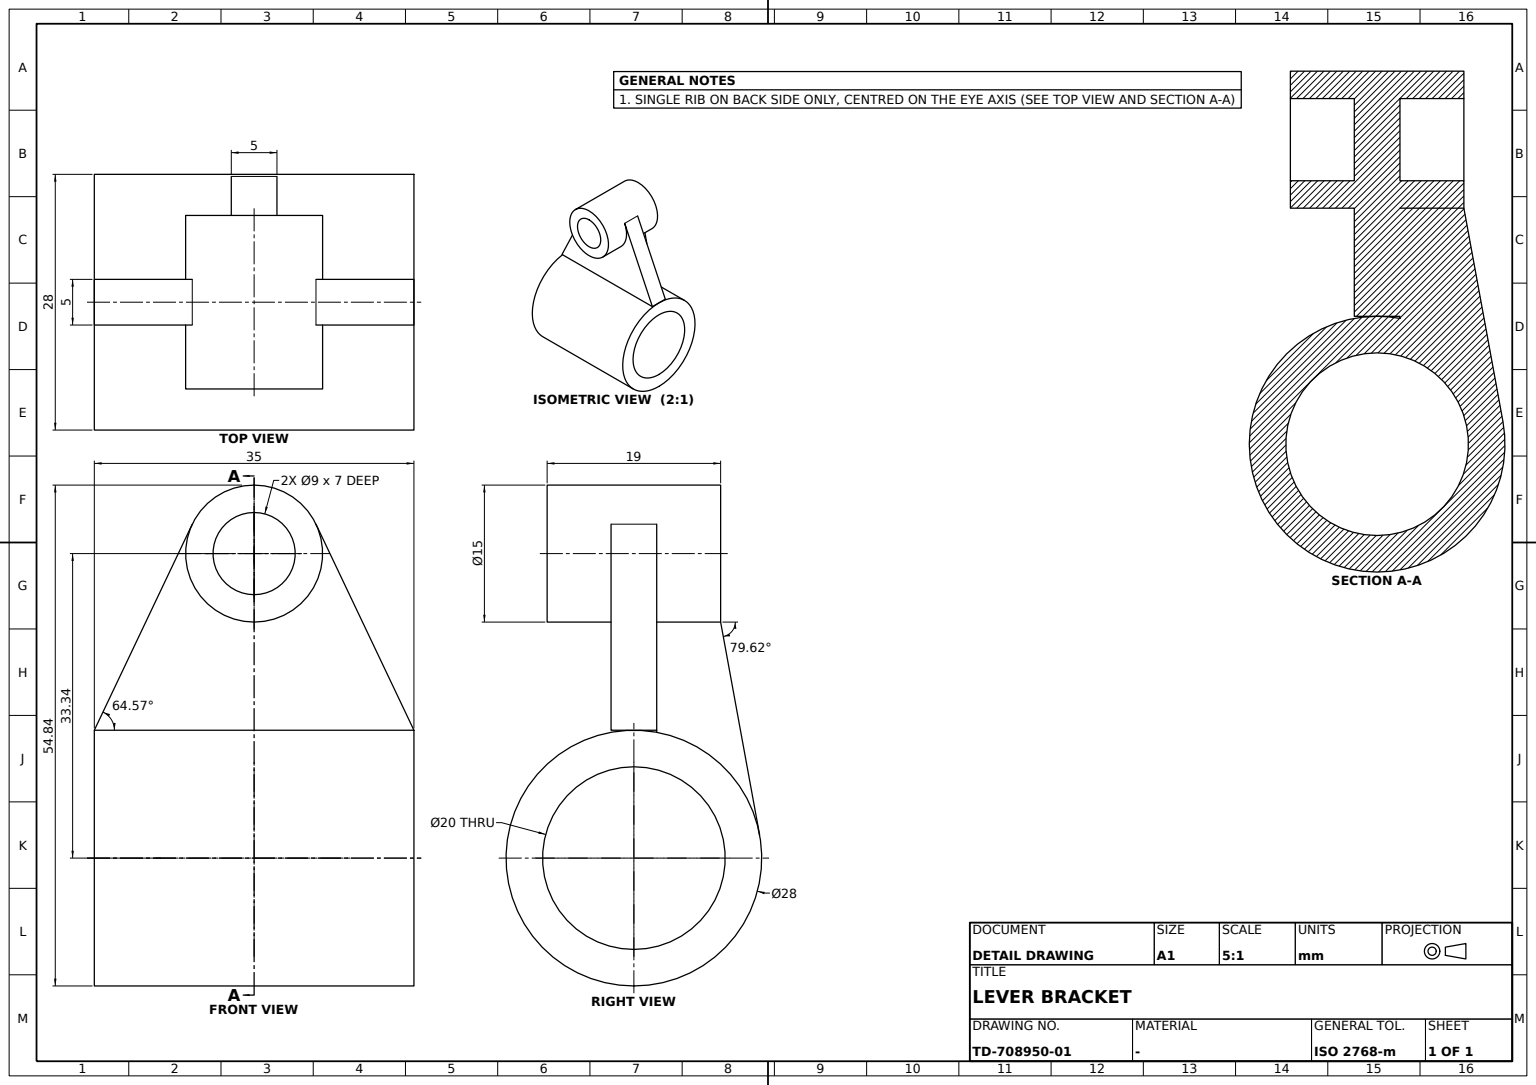
ISO-10303-21;
HEADER;
FILE_DESCRIPTION((''),'2;1');
FILE_NAME('','',(''),(''),'','','');
FILE_SCHEMA(('AUTOMOTIVE_DESIGN'));
ENDSEC;
DATA;
#1=APPLICATION_CONTEXT('');
#2=PRODUCT_CONTEXT('',#1,'mechanical');
#3=PRODUCT('','','',(#2));
#4=PRODUCT_DEFINITION_FORMATION('','',#3);
#5=PRODUCT_DEFINITION_CONTEXT('',#1,'design');
#6=PRODUCT_DEFINITION('','',#4,#5);
#7=PRODUCT_DEFINITION_SHAPE('','',#6);
#8=(LENGTH_UNIT()NAMED_UNIT(*)SI_UNIT(.MILLI.,.METRE.));
#9=(NAMED_UNIT(*)PLANE_ANGLE_UNIT()SI_UNIT($,.RADIAN.));
#10=(NAMED_UNIT(*)SI_UNIT($,.STERADIAN.)SOLID_ANGLE_UNIT());
#11=UNCERTAINTY_MEASURE_WITH_UNIT(LENGTH_MEASURE(0.005),#8,'distance_accuracy_value','');
#12=(GEOMETRIC_REPRESENTATION_CONTEXT(3)GLOBAL_UNCERTAINTY_ASSIGNED_CONTEXT((#11))GLOBAL_UNIT_ASSIGNED_CONTEXT((#8,#9,#10))REPRESENTATION_CONTEXT('',''));
#13=CARTESIAN_POINT('',(0.,2.5,37.842022));
#14=VERTEX_POINT('',#13);
#15=CARTESIAN_POINT('',(0.,2.5,33.342022));
#16=DIRECTION('',(0.,1.,0.));
#17=DIRECTION('',(0.,0.,1.));
#18=AXIS2_PLACEMENT_3D('',#15,#16,#17);
#19=CIRCLE('',#18,4.5);
#20=EDGE_CURVE('',#14,#14,#19,.T.);
#21=ORIENTED_EDGE('',*,*,#20,.F.);
#22=EDGE_LOOP('',(#21));
#23=FACE_BOUND('',#22,.T.);
#24=CARTESIAN_POINT('',(0.,9.5,37.842022));
#25=VERTEX_POINT('',#24);
#26=CARTESIAN_POINT('',(0.,9.5,33.342022));
#27=AXIS2_PLACEMENT_3D('',#26,#16,#17);
#28=CIRCLE('',#27,4.5);
#29=EDGE_CURVE('',#25,#25,#28,.T.);
#30=ORIENTED_EDGE('',*,*,#29,.T.);
#31=EDGE_LOOP('',(#30));
#32=FACE_BOUND('',#31,.T.);
#33=CARTESIAN_POINT('',(0.,0.,33.342022));
#34=DIRECTION('',(-1.,0.,0.));
#35=AXIS2_PLACEMENT_3D('',#33,#16,#34);
#36=CYLINDRICAL_SURFACE('',#35,4.5);
#37=ADVANCED_FACE('',(#23,#32),#36,.F.);
#38=CARTESIAN_POINT('',(17.5,0.,-10.));
#39=VERTEX_POINT('',#38);
#40=CARTESIAN_POINT('',(17.5,0.,0.));
#41=DIRECTION('',(1.,0.,0.));
#42=DIRECTION('',(0.,0.,-1.));
#43=AXIS2_PLACEMENT_3D('',#40,#41,#42);
#44=CIRCLE('',#43,10.);
#45=EDGE_CURVE('',#39,#39,#44,.T.);
#46=ORIENTED_EDGE('',*,*,#45,.T.);
#47=EDGE_LOOP('',(#46));
#48=FACE_BOUND('',#47,.T.);
#49=CARTESIAN_POINT('',(-17.5,0.,-10.));
#50=VERTEX_POINT('',#49);
#51=CARTESIAN_POINT('',(-17.5,0.,0.));
#52=AXIS2_PLACEMENT_3D('',#51,#41,#42);
#53=CIRCLE('',#52,10.);
#54=EDGE_CURVE('',#50,#50,#53,.T.);
#55=ORIENTED_EDGE('',*,*,#54,.F.);
#56=EDGE_LOOP('',(#55));
#57=FACE_BOUND('',#56,.T.);
#58=CARTESIAN_POINT('',(0.,0.,0.));
#59=AXIS2_PLACEMENT_3D('',#58,#41,#16);
#60=CYLINDRICAL_SURFACE('',#59,10.);
#61=ADVANCED_FACE('',(#48,#57),#60,.F.);
#62=CARTESIAN_POINT('',(2.5,2.5,14.));
#63=VERTEX_POINT('',#62);
#64=CARTESIAN_POINT('',(2.5,2.5,13.774977));
#65=VERTEX_POINT('',#64);
#66=CARTESIAN_POINT('',(2.5,2.5,0.));
#67=VECTOR('',#42,1000.);
#68=LINE('',#66,#67);
#69=EDGE_CURVE('',#63,#65,#68,.T.);
#70=ORIENTED_EDGE('',*,*,#69,.F.);
#71=CARTESIAN_POINT('',(-2.5,2.5,14.));
#72=VERTEX_POINT('',#71);
#73=CARTESIAN_POINT('',(0.,2.5,14.));
#74=VECTOR('',#34,1000.);
#75=LINE('',#73,#74);
#76=EDGE_CURVE('',#63,#72,#75,.T.);
#77=ORIENTED_EDGE('',*,*,#76,.T.);
#78=CARTESIAN_POINT('',(-2.5,2.5,13.774977));
#79=VERTEX_POINT('',#78);
#80=CARTESIAN_POINT('',(-2.5,2.5,0.));
#81=LINE('',#80,#67);
#82=EDGE_CURVE('',#72,#79,#81,.T.);
#83=ORIENTED_EDGE('',*,*,#82,.T.);
#84=VECTOR('',#41,1000.);
#85=LINE('',#78,#84);
#86=EDGE_CURVE('',#79,#65,#85,.T.);
#87=ORIENTED_EDGE('',*,*,#86,.T.);
#88=EDGE_LOOP('',(#70,#77,#83,#87));
#89=FACE_BOUND('',#88,.T.);
#90=CARTESIAN_POINT('',(0.,2.5,0.));
#91=AXIS2_PLACEMENT_3D('',#90,#16,#34);
#92=PLANE('',#91);
#93=ADVANCED_FACE('',(#89),#92,.F.);
#94=ORIENTED_EDGE('',*,*,#45,.F.);
#95=EDGE_LOOP('',(#94));
#96=FACE_BOUND('',#95,.T.);
#97=CARTESIAN_POINT('',(17.5,0.,-14.));
#98=VERTEX_POINT('',#97);
#99=CIRCLE('',#43,14.);
#100=EDGE_CURVE('',#98,#98,#99,.T.);
#101=ORIENTED_EDGE('',*,*,#100,.T.);
#102=EDGE_LOOP('',(#101));
#103=FACE_BOUND('',#102,.T.);
#104=AXIS2_PLACEMENT_3D('',#40,#41,#16);
#105=PLANE('',#104);
#106=ADVANCED_FACE('',(#96,#103),#105,.T.);
#107=CARTESIAN_POINT('',(-6.773482,-2.5,36.562261));
#108=VERTEX_POINT('',#107);
#109=CARTESIAN_POINT('',(-6.773482,2.5,36.562261));
#110=VERTEX_POINT('',#109);
#111=CARTESIAN_POINT('',(-6.773482,0.,36.562261));
#112=VECTOR('',#16,1000.);
#113=LINE('',#111,#112);
#114=EDGE_CURVE('',#108,#110,#113,.T.);
#115=ORIENTED_EDGE('',*,*,#114,.T.);
#116=CARTESIAN_POINT('',(-17.5,2.5,14.));
#117=VERTEX_POINT('',#116);
#118=CARTESIAN_POINT('',(-19.702619,2.5,9.366991));
#119=DIRECTION('',(0.429365223,0.,0.903130946));
#120=VECTOR('',#119,1000.);
#121=LINE('',#118,#120);
#122=EDGE_CURVE('',#117,#110,#121,.T.);
#123=ORIENTED_EDGE('',*,*,#122,.F.);
#124=CARTESIAN_POINT('',(-17.5,-2.5,14.));
#125=VERTEX_POINT('',#124);
#126=CARTESIAN_POINT('',(-17.5,0.,14.));
#127=LINE('',#126,#112);
#128=EDGE_CURVE('',#125,#117,#127,.T.);
#129=ORIENTED_EDGE('',*,*,#128,.F.);
#130=CARTESIAN_POINT('',(-19.702619,-2.5,9.366991));
#131=LINE('',#130,#120);
#132=EDGE_CURVE('',#125,#108,#131,.T.);
#133=ORIENTED_EDGE('',*,*,#132,.T.);
#134=EDGE_LOOP('',(#115,#123,#129,#133));
#135=FACE_BOUND('',#134,.T.);
#136=DIRECTION('',(-0.903130946,0.,0.429365223));
#137=AXIS2_PLACEMENT_3D('',#126,#136,#119);
#138=PLANE('',#137);
#139=ADVANCED_FACE('',(#135),#138,.T.);
#140=ORIENTED_EDGE('',*,*,#76,.F.);
#141=CARTESIAN_POINT('',(17.5,2.5,14.));
#142=VERTEX_POINT('',#141);
#143=EDGE_CURVE('',#142,#63,#75,.T.);
#144=ORIENTED_EDGE('',*,*,#143,.F.);
#145=CARTESIAN_POINT('',(17.5,-2.5,14.));
#146=VERTEX_POINT('',#145);
#147=CARTESIAN_POINT('',(17.5,0.,14.));
#148=LINE('',#147,#112);
#149=EDGE_CURVE('',#146,#142,#148,.T.);
#150=ORIENTED_EDGE('',*,*,#149,.F.);
#151=CARTESIAN_POINT('',(0.,-2.5,14.));
#152=LINE('',#151,#74);
#153=EDGE_CURVE('',#146,#125,#152,.T.);
#154=ORIENTED_EDGE('',*,*,#153,.T.);
#155=ORIENTED_EDGE('',*,*,#128,.T.);
#156=EDGE_CURVE('',#72,#117,#75,.T.);
#157=ORIENTED_EDGE('',*,*,#156,.F.);
#158=EDGE_LOOP('',(#140,#144,#150,#154,#155,#157));
#159=FACE_BOUND('',#158,.T.);
#160=AXIS2_PLACEMENT_3D('',#147,#42,#34);
#161=PLANE('',#160);
#162=ADVANCED_FACE('',(#159),#161,.T.);
#163=ORIENTED_EDGE('',*,*,#143,.T.);
#164=CARTESIAN_POINT('',(2.5,2.5,25.842022));
#165=VERTEX_POINT('',#164);
#166=EDGE_CURVE('',#165,#63,#68,.T.);
#167=ORIENTED_EDGE('',*,*,#166,.F.);
#168=CARTESIAN_POINT('',(0.,2.5,25.842022));
#169=VERTEX_POINT('',#168);
#170=LINE('',#168,#84);
#171=EDGE_CURVE('',#169,#165,#170,.T.);
#172=ORIENTED_EDGE('',*,*,#171,.F.);
#173=CARTESIAN_POINT('',(6.773482,2.5,36.562261));
#174=VERTEX_POINT('',#173);
#175=CIRCLE('',#18,7.5);
#176=EDGE_CURVE('',#174,#169,#175,.T.);
#177=ORIENTED_EDGE('',*,*,#176,.F.);
#178=CARTESIAN_POINT('',(19.702619,2.5,9.366991));
#179=DIRECTION('',(0.429365223,0.,-0.903130946));
#180=VECTOR('',#179,1000.);
#181=LINE('',#178,#180);
#182=EDGE_CURVE('',#174,#142,#181,.T.);
#183=ORIENTED_EDGE('',*,*,#182,.T.);
#184=EDGE_LOOP('',(#163,#167,#172,#177,#183));
#185=FACE_BOUND('',#184,.T.);
#186=ADVANCED_FACE('',(#185),#92,.T.);
#187=CARTESIAN_POINT('',(0.,-2.5,37.842022));
#188=VERTEX_POINT('',#187);
#189=CARTESIAN_POINT('',(0.,-2.5,33.342022));
#190=AXIS2_PLACEMENT_3D('',#189,#16,#17);
#191=CIRCLE('',#190,4.5);
#192=EDGE_CURVE('',#188,#188,#191,.T.);
#193=ORIENTED_EDGE('',*,*,#192,.F.);
#194=EDGE_LOOP('',(#193));
#195=FACE_BOUND('',#194,.T.);
#196=CARTESIAN_POINT('',(0.,-2.5,0.));
#197=AXIS2_PLACEMENT_3D('',#196,#16,#34);
#198=PLANE('',#197);
#199=ADVANCED_FACE('',(#195),#198,.F.);
#200=ORIENTED_EDGE('',*,*,#82,.F.);
#201=CARTESIAN_POINT('',(-2.5,2.5,25.842022));
#202=VERTEX_POINT('',#201);
#203=EDGE_CURVE('',#202,#72,#81,.T.);
#204=ORIENTED_EDGE('',*,*,#203,.F.);
#205=CARTESIAN_POINT('',(-2.5,9.5,25.842022));
#206=VERTEX_POINT('',#205);
#207=CARTESIAN_POINT('',(-2.5,0.,25.842022));
#208=LINE('',#207,#112);
#209=EDGE_CURVE('',#202,#206,#208,.T.);
#210=ORIENTED_EDGE('',*,*,#209,.T.);
#211=CARTESIAN_POINT('',(-2.5,13.770949,2.522093));
#212=VERTEX_POINT('',#211);
#213=DIRECTION('',(0.,0.180149495,-0.983639243));
#214=VECTOR('',#213,1000.);
#215=LINE('',#211,#214);
#216=EDGE_CURVE('',#206,#212,#215,.T.);
#217=ORIENTED_EDGE('',*,*,#216,.T.);
#218=CARTESIAN_POINT('',(-2.5,0.,0.));
#219=AXIS2_PLACEMENT_3D('',#218,#41,#42);
#220=CIRCLE('',#219,14.);
#221=EDGE_CURVE('',#212,#79,#220,.T.);
#222=ORIENTED_EDGE('',*,*,#221,.T.);
#223=EDGE_LOOP('',(#200,#204,#210,#217,#222));
#224=FACE_BOUND('',#223,.T.);
#225=AXIS2_PLACEMENT_3D('',#218,#41,#16);
#226=PLANE('',#225);
#227=ADVANCED_FACE('',(#224),#226,.F.);
#228=ORIENTED_EDGE('',*,*,#20,.T.);
#229=EDGE_LOOP('',(#228));
#230=FACE_BOUND('',#229,.T.);
#231=ADVANCED_FACE('',(#230),#92,.T.);
#232=CARTESIAN_POINT('',(-17.5,0.,-14.));
#233=VERTEX_POINT('',#232);
#234=CIRCLE('',#52,14.);
#235=EDGE_CURVE('',#233,#233,#234,.T.);
#236=ORIENTED_EDGE('',*,*,#235,.T.);
#237=EDGE_LOOP('',(#236));
#238=FACE_BOUND('',#237,.T.);
#239=ORIENTED_EDGE('',*,*,#100,.F.);
#240=EDGE_LOOP('',(#239));
#241=FACE_BOUND('',#240,.T.);
#242=ORIENTED_EDGE('',*,*,#221,.F.);
#243=CARTESIAN_POINT('',(2.5,13.770949,2.522093));
#244=VERTEX_POINT('',#243);
#245=CARTESIAN_POINT('',(0.,13.770949,2.522093));
#246=LINE('',#245,#84);
#247=EDGE_CURVE('',#212,#244,#246,.T.);
#248=ORIENTED_EDGE('',*,*,#247,.T.);
#249=CARTESIAN_POINT('',(2.5,0.,0.));
#250=AXIS2_PLACEMENT_3D('',#249,#41,#42);
#251=CIRCLE('',#250,14.);
#252=EDGE_CURVE('',#244,#65,#251,.T.);
#253=ORIENTED_EDGE('',*,*,#252,.T.);
#254=ORIENTED_EDGE('',*,*,#86,.F.);
#255=EDGE_LOOP('',(#242,#248,#253,#254));
#256=FACE_BOUND('',#255,.T.);
#257=CYLINDRICAL_SURFACE('',#59,14.);
#258=ADVANCED_FACE('',(#238,#241,#256),#257,.T.);
#259=CARTESIAN_POINT('',(0.,-9.5,40.842022));
#260=VERTEX_POINT('',#259);
#261=CARTESIAN_POINT('',(0.,-9.5,33.342022));
#262=AXIS2_PLACEMENT_3D('',#261,#16,#17);
#263=CIRCLE('',#262,7.5);
#264=EDGE_CURVE('',#260,#260,#263,.T.);
#265=ORIENTED_EDGE('',*,*,#264,.F.);
#266=EDGE_LOOP('',(#265));
#267=FACE_BOUND('',#266,.T.);
#268=CARTESIAN_POINT('',(0.,-9.5,37.842022));
#269=VERTEX_POINT('',#268);
#270=CIRCLE('',#262,4.5);
#271=EDGE_CURVE('',#269,#269,#270,.T.);
#272=ORIENTED_EDGE('',*,*,#271,.T.);
#273=EDGE_LOOP('',(#272));
#274=FACE_BOUND('',#273,.T.);
#275=CARTESIAN_POINT('',(0.,-9.5,0.));
#276=AXIS2_PLACEMENT_3D('',#275,#16,#34);
#277=PLANE('',#276);
#278=ADVANCED_FACE('',(#267,#274),#277,.F.);
#279=ORIENTED_EDGE('',*,*,#176,.T.);
#280=EDGE_CURVE('',#169,#110,#175,.T.);
#281=ORIENTED_EDGE('',*,*,#280,.T.);
#282=ORIENTED_EDGE('',*,*,#114,.F.);
#283=CARTESIAN_POINT('',(6.773482,-2.5,36.562261));
#284=VERTEX_POINT('',#283);
#285=CIRCLE('',#190,7.5);
#286=EDGE_CURVE('',#284,#108,#285,.T.);
#287=ORIENTED_EDGE('',*,*,#286,.F.);
#288=CARTESIAN_POINT('',(6.773482,0.,36.562261));
#289=LINE('',#288,#112);
#290=EDGE_CURVE('',#284,#174,#289,.T.);
#291=ORIENTED_EDGE('',*,*,#290,.T.);
#292=EDGE_LOOP('',(#279,#281,#282,#287,#291));
#293=FACE_BOUND('',#292,.T.);
#294=CARTESIAN_POINT('',(0.,9.5,40.842022));
#295=VERTEX_POINT('',#294);
#296=CIRCLE('',#27,7.5);
#297=EDGE_CURVE('',#295,#295,#296,.T.);
#298=ORIENTED_EDGE('',*,*,#297,.F.);
#299=EDGE_LOOP('',(#298));
#300=FACE_BOUND('',#299,.T.);
#301=ORIENTED_EDGE('',*,*,#264,.T.);
#302=EDGE_LOOP('',(#301));
#303=FACE_BOUND('',#302,.T.);
#304=CYLINDRICAL_SURFACE('',#35,7.5);
#305=ADVANCED_FACE('',(#293,#300,#303),#304,.T.);
#306=ORIENTED_EDGE('',*,*,#122,.T.);
#307=ORIENTED_EDGE('',*,*,#280,.F.);
#308=EDGE_CURVE('',#202,#169,#170,.T.);
#309=ORIENTED_EDGE('',*,*,#308,.F.);
#310=ORIENTED_EDGE('',*,*,#203,.T.);
#311=ORIENTED_EDGE('',*,*,#156,.T.);
#312=EDGE_LOOP('',(#306,#307,#309,#310,#311));
#313=FACE_BOUND('',#312,.T.);
#314=ADVANCED_FACE('',(#313),#92,.T.);
#315=ORIENTED_EDGE('',*,*,#29,.F.);
#316=EDGE_LOOP('',(#315));
#317=FACE_BOUND('',#316,.T.);
#318=ORIENTED_EDGE('',*,*,#297,.T.);
#319=EDGE_LOOP('',(#318));
#320=FACE_BOUND('',#319,.T.);
#321=CARTESIAN_POINT('',(0.,9.5,0.));
#322=AXIS2_PLACEMENT_3D('',#321,#16,#34);
#323=PLANE('',#322);
#324=ADVANCED_FACE('',(#317,#320),#323,.T.);
#325=ORIENTED_EDGE('',*,*,#171,.T.);
#326=CARTESIAN_POINT('',(2.5,9.5,25.842022));
#327=VERTEX_POINT('',#326);
#328=CARTESIAN_POINT('',(2.5,0.,25.842022));
#329=LINE('',#328,#112);
#330=EDGE_CURVE('',#165,#327,#329,.T.);
#331=ORIENTED_EDGE('',*,*,#330,.T.);
#332=CARTESIAN_POINT('',(0.,9.5,25.842022));
#333=LINE('',#332,#84);
#334=EDGE_CURVE('',#206,#327,#333,.T.);
#335=ORIENTED_EDGE('',*,*,#334,.F.);
#336=ORIENTED_EDGE('',*,*,#209,.F.);
#337=ORIENTED_EDGE('',*,*,#308,.T.);
#338=EDGE_LOOP('',(#325,#331,#335,#336,#337));
#339=FACE_BOUND('',#338,.T.);
#340=AXIS2_PLACEMENT_3D('',#168,#42,#16);
#341=PLANE('',#340);
#342=ADVANCED_FACE('',(#339),#341,.F.);
#343=LINE('',#243,#214);
#344=EDGE_CURVE('',#327,#244,#343,.T.);
#345=ORIENTED_EDGE('',*,*,#344,.T.);
#346=ORIENTED_EDGE('',*,*,#247,.F.);
#347=ORIENTED_EDGE('',*,*,#216,.F.);
#348=ORIENTED_EDGE('',*,*,#334,.T.);
#349=EDGE_LOOP('',(#345,#346,#347,#348));
#350=FACE_BOUND('',#349,.T.);
#351=DIRECTION('',(0.,-0.983639243,-0.180149495));
#352=AXIS2_PLACEMENT_3D('',#332,#351,#213);
#353=PLANE('',#352);
#354=ADVANCED_FACE('',(#350),#353,.F.);
#355=ORIENTED_EDGE('',*,*,#54,.T.);
#356=EDGE_LOOP('',(#355));
#357=FACE_BOUND('',#356,.T.);
#358=ORIENTED_EDGE('',*,*,#235,.F.);
#359=EDGE_LOOP('',(#358));
#360=FACE_BOUND('',#359,.T.);
#361=AXIS2_PLACEMENT_3D('',#51,#41,#16);
#362=PLANE('',#361);
#363=ADVANCED_FACE('',(#357,#360),#362,.F.);
#364=ORIENTED_EDGE('',*,*,#330,.F.);
#365=ORIENTED_EDGE('',*,*,#166,.T.);
#366=ORIENTED_EDGE('',*,*,#69,.T.);
#367=ORIENTED_EDGE('',*,*,#252,.F.);
#368=ORIENTED_EDGE('',*,*,#344,.F.);
#369=EDGE_LOOP('',(#364,#365,#366,#367,#368));
#370=FACE_BOUND('',#369,.T.);
#371=AXIS2_PLACEMENT_3D('',#249,#41,#16);
#372=PLANE('',#371);
#373=ADVANCED_FACE('',(#370),#372,.T.);
#374=ORIENTED_EDGE('',*,*,#149,.T.);
#375=ORIENTED_EDGE('',*,*,#182,.F.);
#376=ORIENTED_EDGE('',*,*,#290,.F.);
#377=CARTESIAN_POINT('',(19.702619,-2.5,9.366991));
#378=LINE('',#377,#180);
#379=EDGE_CURVE('',#284,#146,#378,.T.);
#380=ORIENTED_EDGE('',*,*,#379,.T.);
#381=EDGE_LOOP('',(#374,#375,#376,#380));
#382=FACE_BOUND('',#381,.T.);
#383=DIRECTION('',(0.903130946,0.,0.429365223));
#384=AXIS2_PLACEMENT_3D('',#288,#383,#179);
#385=PLANE('',#384);
#386=ADVANCED_FACE('',(#382),#385,.T.);
#387=ORIENTED_EDGE('',*,*,#192,.T.);
#388=EDGE_LOOP('',(#387));
#389=FACE_BOUND('',#388,.T.);
#390=ORIENTED_EDGE('',*,*,#271,.F.);
#391=EDGE_LOOP('',(#390));
#392=FACE_BOUND('',#391,.T.);
#393=ADVANCED_FACE('',(#389,#392),#36,.F.);
#394=ORIENTED_EDGE('',*,*,#132,.F.);
#395=ORIENTED_EDGE('',*,*,#153,.F.);
#396=ORIENTED_EDGE('',*,*,#379,.F.);
#397=ORIENTED_EDGE('',*,*,#286,.T.);
#398=EDGE_LOOP('',(#394,#395,#396,#397));
#399=FACE_BOUND('',#398,.T.);
#400=ADVANCED_FACE('',(#399),#198,.F.);
#401=CLOSED_SHELL('',(#37,#61,#93,#106,#139,#162,#186,#199,#227,#231,#258,#278,#305,#314,#324,#342,#354,#363,#373,#386,#393,#400));
#402=MANIFOLD_SOLID_BREP('',#401);
#403=ADVANCED_BREP_SHAPE_REPRESENTATION('',(#402),#12);
#404=SHAPE_DEFINITION_REPRESENTATION(#7,#403);
ENDSEC;
END-ISO-10303-21;
